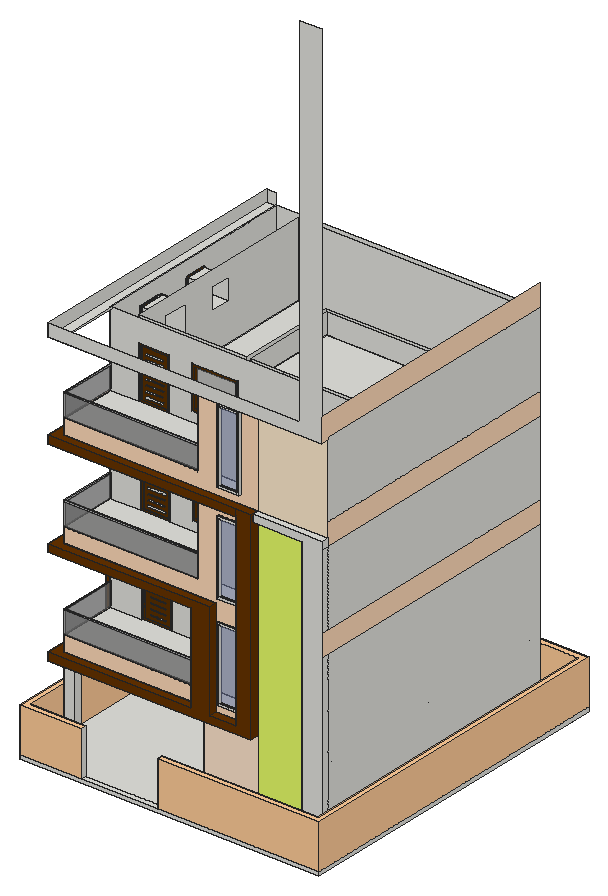
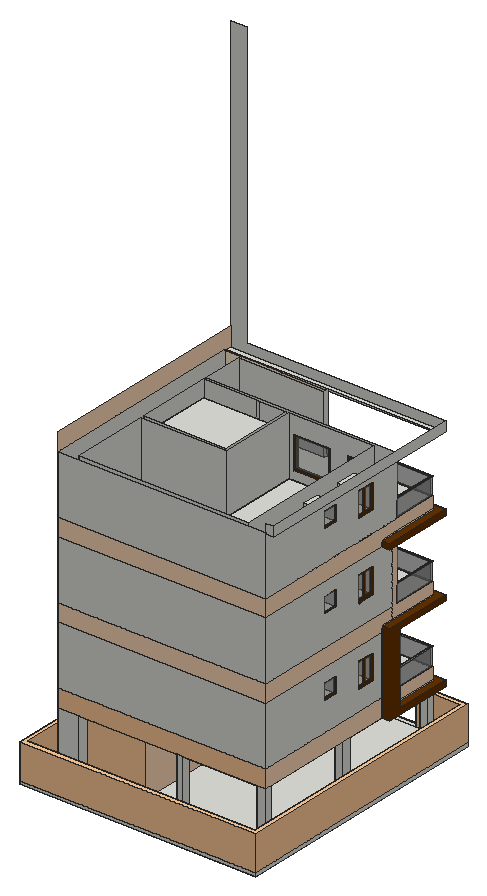
# SketchUp Ruby script. Lengths in inches.
U = 1.inch
M = Sketchup.active_model
def pt(a) = Geom::Point3d.new(a.map { |v| v * U })
def face(e, loops, mat)
  f = e.add_face(loops[0].map { |a| pt(a) })
  loops[1..].each { |l| e.add_face(l.map { |a| pt(a) }).erase! }
  f.material = f.back_material = mat if mat
  f
end
# faces: each face lists its corners as indices into pts; further lists are holes
def faces(e, pts, list, mat = nil) = list.each { |f| face(e, (f[0].is_a?(Array) ? f : [f]).map { |l| l.map { |i| pts[i] } }, mat) }
# xy, xz, yz: faces in a plane at the given z, y or x. An outline is a flat list of corners, or four numbers for a rectangle; further outlines are holes
def ring(l) = l.size == 4 ? [[l[0], l[1]], [l[2], l[1]], [l[2], l[3]], [l[0], l[3]]] : l.each_slice(2).to_a
def flat(e, list, mat, &to3) = list.each { |f| face(e, (f[0].is_a?(Array) ? f : [f]).map { |l| ring(l).map { |u, v| to3.(u, v) } }, mat) }
def xy(e, z, list, mat = nil) = flat(e, list, mat) { |x, y| [x, y, z] }
def xz(e, y, list, mat = nil) = flat(e, list, mat) { |x, z| [x, y, z] }
def yz(e, x, list, mat = nil) = flat(e, list, mat) { |y, z| [x, y, z] }
def lines(e, pts, list) = list.each { |a, b| e.add_line(pt(pts[a]), pt(pts[b])) }
# prism: a flat outline (further loops are holes) pulled along v
def prism(e, loops, v, mat = nil)
  f = face(e, loops, mat); d = Geom::Vector3d.new(v.map { |x| x * U })
  f.pushpull(f.normal.samedirection?(d) ? d.length : -d.length)
end
def box(e, o, s, mat = nil) = prism(e, [[o, [o[0] + s[0], o[1], o[2]], [o[0] + s[0], o[1] + s[1], o[2]], [o[0], o[1] + s[1], o[2]]]], [0, 0, s[2]], mat)
def at(x, y, z, deg = 0) = Geom::Transformation.translation(pt([x, y, z])) * Geom::Transformation.rotation(ORIGIN, Z_AXIS, deg.degrees)
def axes(o, x, y, z) = Geom::Transformation.new([*x, 0, *y, 0, *z, 0, *pt(o).to_a, 1])
def part(name) = M.definitions.add(name)
# library, detail: a bought-in or finely detailed component or shape, given as its bounding box
def library(name, o, s) = part(name).tap { |d| box(d.entities, o, s) }
def detail(e, o, s) = box(e.add_group.entities, o, s)
def put(e, d, t, mat = nil) = e.add_instance(d, t).tap { |i| i.material = mat if mat }
def group(e, t, mat = nil) = e.add_group.tap { |g| g.transformation = t; g.material = mat if mat }.entities
root = M.entities
M.materials.add("[0027_PeachPuff]").color = [255, 218, 185]
M.materials.add("[0029_BlanchedAlmond]").color = [255, 235, 205]
M.materials.add("[Aluminum]").color = [179, 179, 179]
M.materials.add("[Color A08]").color = [89, 48, 0]
M.materials.add("[Color C01]").color = [255, 229, 204]
M.materials.add("[Color C02]").color = [255, 204, 153]
M.materials.add("[Color C08]").color = [102, 51, 0]
M.materials.add("[Color M00]").color = [255, 255, 255]
M.materials.add("[Rectangles Running 4x1]").color = [231, 255, 106]
M.materials.add("[Translucent Glass Gray]").color = [128, 128, 128]
M.materials["[Translucent Glass Gray]"].alpha = 0.5
M.materials.add("[Translucent Glass Sky Reflection]").color = [126, 138, 183]
M.materials["[Translucent Glass Sky Reflection]"].alpha = 0.52
c1 = part("Group\#2")
xy(c1.entities,0,[[0,0,48,6.0625]],"[Color A08]")
xy(c1.entities,2.37,[[2.37,2.1875,45.63,6.0625]])
xy(c1.entities,2.37,[[2.37,0,45.63,2.1875]],"[Color A08]")
xy(c1.entities,81.63,[[2.37,2.1875,45.63,6.0625]])
xy(c1.entities,81.63,[[2.37,0,45.63,2.1875]],"[Color A08]")
xy(c1.entities,84,[[0,0,48,6.0625]],"[Color A08]")
xz(c1.entities,0,[[[0,0,48,84],[2.37,2.37,45.63,81.63]]],"[Color A08]")
xz(c1.entities,2.1875,[[9.64,6.54,37.83,9.91],[9.64,15.35,37.83,18.72],[9.64,24.16,37.83,27.54],[9.64,32.97,37.83,36.35],[9.64,41.79,37.83,45.16],
  [9.64,50.6,37.83,53.97],[9.64,59.41,37.83,62.79],[9.64,68.22,37.83,71.6]])
xz(c1.entities,2.1875,[[[2.37,2.37,45.63,81.63],[9.64,68.22,37.83,71.6],[9.64,59.41,37.83,62.79],[9.64,50.6,37.83,53.97],[9.64,41.79,37.83,45.16],[9.64,32.97,37.83,36.35],[9.64,24.16,37.83,27.54],[9.64,15.35,37.83,18.72],[9.64,6.54,37.83,9.91]]],"[Color A08]")
xz(c1.entities,6.0625,[[[0,0,48,84],[2.37,2.37,45.63,81.63]],[2.37,2.37,45.63,81.63]],"[Color A08]")
yz(c1.entities,0,[[0,0,6.0625,84]],"[Color A08]")
yz(c1.entities,2.37,[[2.1875,2.37,6.0625,81.63]])
yz(c1.entities,2.37,[[0,2.37,2.1875,81.63]],"[Color A08]")
yz(c1.entities,45.63,[[2.1875,2.37,6.0625,81.63]])
yz(c1.entities,45.63,[[0,2.37,2.1875,81.63]],"[Color A08]")
yz(c1.entities,48,[[0,0,6.0625,84]],"[Color A08]")
c2 = part("Group\#1")
xy(c2.entities,0,[[0,0,54.25,4.125]],"[Color A08]")
xy(c2.entities,2.45,[[2.45,0,51.8,4.125]],"[Color A08]")
xy(c2.entities,43.87,[[2.45,0,51.8,4.125]],"[Color A08]")
xy(c2.entities,46.3125,[[0,0,54.25,4.125]],"[Color A08]")
xz(c2.entities,0,[[[0,0,54.25,46.3125],[2.45,2.45,51.8,43.87]]],"[Color A08]")
xz(c2.entities,4.125,[[[0,0,54.25,46.3125],[2.45,2.45,51.8,43.87]]],"[Color A08]")
xz(c2.entities,4.125,[[2.45,2.45,51.8,43.87]],"[Translucent Glass Gray]")
yz(c2.entities,0,[[0,0,4.125,46.3125]],"[Color A08]")
yz(c2.entities,2.45,[[0,2.45,4.125,43.87]],"[Color A08]")
yz(c2.entities,51.8,[[0,2.45,4.125,43.87]],"[Color A08]")
yz(c2.entities,54.25,[[0,0,4.125,46.3125]],"[Color A08]")
c3 = part("Group\#3")
xy(c3.entities,0,[[0,0,1.5,39.25],[1.5,0,2.8125,39.25]],"[Color A08]")
xy(c3.entities,3.22,[[0,3.22,1.5,19.0625],[1.5,3.22,2.8125,19.0625],[1.5,19.0625,2.8125,22.29],[0,22.29,1.5,36.03],[1.5,22.29,2.8125,36.03]],"[Color A08]")
xy(c3.entities,36.03,[[0,3.22,1.5,19.0625],[1.5,3.22,2.8125,19.0625],[0,19.0625,1.5,22.29],[1.5,19.0625,2.8125,22.29],[0,22.29,1.5,36.03],
  [1.5,22.29,2.8125,36.03]],"[Color A08]")
xy(c3.entities,39.25,[[0,0,1.5,39.25],[1.5,0,2.8125,39.25]],"[Color A08]")
xz(c3.entities,0,[[0,0,1.5,39.25],[1.5,0,2.8125,39.25]],"[Color A08]")
xz(c3.entities,3.22,[[0,3.22,1.5,36.03],[1.5,3.22,2.8125,36.03]],"[Color A08]")
xz(c3.entities,19.0625,[[0,3.22,1.5,36.03],[1.5,3.22,2.8125,36.03]],"[Color A08]")
xz(c3.entities,22.29,[[0,3.22,1.5,36.03],[1.5,3.22,2.8125,36.03]],"[Color A08]")
xz(c3.entities,36.03,[[0,3.22,1.5,36.03],[1.5,3.22,2.8125,36.03]],"[Color A08]")
xz(c3.entities,39.25,[[0,0,1.5,39.25],[1.5,0,2.8125,39.25]],"[Color A08]")
yz(c3.entities,0,[[[0,0,39.25,39.25],[3.22,3.22,19.0625,36.03],[22.29,3.22,36.03,36.03]]],"[Color A08]")
yz(c3.entities,1.5,[[[0,0,39.25,39.25],[3.22,3.22,36.03,36.03]],[19.0625,3.22,22.29,36.03]],"[Color A08]")
yz(c3.entities,1.5,[[3.22,3.22,19.0625,36.03],[22.29,3.22,36.03,36.03]],"[Translucent Glass Gray]")
yz(c3.entities,2.8125,[[[0,0,39.25,39.25],[3.22,3.22,36.03,36.03]],[19.0625,3.22,22.29,36.03]],"[Color A08]")
c4 = part("Group\#4")
xy(c4.entities,0,[[0,0,1.5,39.25],[1.5,0,2.8125,39.25]],"[Color A08]")
xy(c4.entities,3.22,[[0,3.22,1.5,36.03],[1.5,3.22,2.8125,36.03]],"[Color A08]")
xy(c4.entities,36.03,[[0,3.22,1.5,36.03],[1.5,3.22,2.8125,36.03]],"[Color A08]")
xy(c4.entities,39.25,[[0,0,1.5,39.25],[1.5,0,2.8125,39.25]],"[Color A08]")
xz(c4.entities,0,[[0,0,1.5,39.25],[1.5,0,2.8125,39.25]],"[Color A08]")
xz(c4.entities,3.22,[[0,3.22,1.5,36.03],[1.5,3.22,2.8125,36.03]],"[Color A08]")
xz(c4.entities,36.03,[[0,3.22,1.5,36.03],[1.5,3.22,2.8125,36.03]],"[Color A08]")
xz(c4.entities,39.25,[[0,0,1.5,39.25],[1.5,0,2.8125,39.25]],"[Color A08]")
yz(c4.entities,0,[[[0,0,39.25,39.25],[3.22,3.22,36.03,36.03]]],"[Color A08]")
yz(c4.entities,1.5,[[[0,0,39.25,39.25],[3.22,3.22,36.03,36.03]]],"[Color A08]")
yz(c4.entities,1.5,[[3.22,3.22,36.03,36.03]],"[Translucent Glass Gray]")
yz(c4.entities,2.8125,[[[0,0,39.25,39.25],[3.22,3.22,36.03,36.03]]],"[Color A08]")
xy(root,0,[[0,0,480,540]],"[Color M00]")
xy(root,6,[[0,0,0,540,480,540,480,0,220.15,0,220.15,9,471,9,471,531,9,531,9,9,98.15,9,98.15,0],[98.15,0,220.15,9],[[9,9,471,531],[414.23,46.6875,414.23,57,249.82,57,249.82,63,417,63,417,251.76,287.75,251.76,287.75,461.375,406.24,461.375,406.24,483,448.4375,483,448.4375,46.6875],[24.5,270.1,42.53,286.06],[24.5,57,42.53,69.13],[24.5,471.06,42.53,483],[193.7,468.4375,207.02,483]],[414.23,46.6875,448.4375,57],[24.5,57,42.53,69.13],
  [249.82,57,249.82,63,417,63,417,251.76,448.4375,251.76,448.4375,57],[[287.75,251.76,448.4375,461.375],[293.77,257.79,417,374.99]],[293.77,257.79,417,374.99],[24.5,270.1,42.53,286.06],[406.24,461.375,448.4375,483],
  [193.7,468.4375,207.02,483],[24.5,471.06,42.53,483]])
xy(root,78,[[0,0,98.15,0,98.15,9,9,9,9,531,471,531,471,9,220.15,9,220.15,0,480,0,480,540,0,540]],"[Color C02]")
xy(root,120,[[293.77,257.79,417,374.99]])
xy(root,126,[[24.5,57,42.53,69.13],[42.53,57,42.53,69.13,24.5,69.13,24.5,270.1,42.53,270.1,42.53,286.06,24.5,286.06,24.5,471.06,42.53,471.06,42.53,483,193.7,483,193.7,468.4375,207.02,468.4375,207.02,483,406.24,483,406.24,461.375,287.75,461.375,287.75,251.76,417,251.76,417,63,249.82,63,249.82,57],[287.75,251.76,293.77,461.375],[293.77,251.76,410.98,257.79],[293.77,257.79,417,374.99],
  [24.5,270.1,42.53,286.06],[293.77,374.99,302.09,461.375],[302.09,374.99,410.98,461.375],[410.98,374.99,417,461.375],[406.24,461.375,410.98,483],
  [410.98,461.375,417,483],[193.7,468.4375,207.02,483],[24.5,471.06,42.53,483]])
xy(root,126,[[9.1875,43.625,9.1875,69.13,24.5,69.13,24.5,57,335.42,57,335.42,43.625],[9.1875,69.13,24.5,187.1]],"[Color C08]")
xy(root,138,[[9.1875,43.625,239.3125,43.625,239.3125,57,24.5,57,24.5,160.8,9.1875,160.8],[268.87,43.625,310.94,57]],"[Color C08]")
xy(root,149.86,[[273.13,54,307.66,57]])
xy(root,152.91,[[276.18,54,304.61,57]])
xy(root,162,[[24.5,57,24.5,149.375,26.5,149.375,26.5,59,239.3125,59,239.3125,57],[26.5,59,239.3125,59,239.3125,66,414,66,414,149.375,123.74,149.375,123.74,155.375,75.74,155.375,75.74,149.375,26.5,149.375],[66,155.375,239.3125,155.375,239.3125,314.6875,414,314.6875,414,474,66,474],[245.3125,155.375,414,308.6875]])
xy(root,179.21,[[157.83,149.375,231.58,155.375]])
xy(root,198,[[24.5,57,24.5,149.375,26.5,149.375,26.5,59,239.3125,59,239.3125,57]],"[Aluminum]")
xy(root,200,[[24.5,57,239.3125,57,239.3125,59,26.5,59,26.5,149.375,24.5,149.375]],"[Aluminum]")
xy(root,202.95,[[24.5,208.14,66,249.33]])
xy(root,220.36,[[24.5,301.46,66,335.96]])
xy(root,246,[[75.74,149.375,123.74,155.375]])
xy(root,247.4,[[157.83,149.375,231.58,155.375]])
xy(root,254.86,[[24.5,301.46,66,335.96]])
xy(root,256.82,[[24.5,208.14,66,249.33]])
xy(root,265.97,[[276.18,54,277.97,57],[277.97,54,280.16,57],[280.16,54,304.61,57]])
xy(root,269.02,[[273.13,54,307.66,57]])
xy(root,282,[[24.5,57,24.5,149.375,414,149.375,414,66,239.3125,66,239.3125,57]])
xy(root,282,[[9.1875,43.625,9.1875,160.8,24.5,160.8,24.5,57,239.3125,57,239.3125,43.625]],"[Color C08]")
xy(root,294,[[9.1875,43.625,268.87,43.625,268.87,57,24.5,57,24.5,187.1,9.1875,187.1]],"[Color C08]")
xy(root,303.05,[[273.13,54,307.66,57]])
xy(root,306.1,[[276.18,54,277.97,57],[277.97,54,304.61,57]])
xy(root,312,[[66,155.375,66,474,414,474,414,314.6875,239.3125,314.6875,239.3125,155.375]])
xy(root,318,[[24.5,57,24.5,149.375,26.5,149.375,26.5,59,239.3125,59,239.3125,57],[26.5,59,239.3125,59,239.3125,66,414,66,414,149.375,121.24,149.375,121.24,155.375,73.24,155.375,73.24,149.375,26.5,149.375],[121.24,149.375,414,155.375],[66,155.375,239.3125,155.375,239.3125,314.6875,414,314.6875,414,474,66,474],[245.3125,155.375,414,308.6875]])
xy(root,325.5625,[[245.3125,155.375,414,308.6875]])
xy(root,332.27,[[156.77,149.375,230.52,155.375]])
xy(root,354,[[24.5,57,24.5,149.375,26.5,149.375,26.5,59,239.3125,59,239.3125,57]],"[Aluminum]")
xy(root,356,[[24.5,57,239.3125,57,239.3125,59,26.5,59,26.5,149.375,24.5,149.375]],"[Aluminum]")
xy(root,360.82,[[24.5,208.14,66,249.33]])
xy(root,378.92,[[24.5,301.46,66,335.96]])
xy(root,400.46,[[156.77,149.375,230.52,155.375]])
xy(root,402,[[73.24,149.375,121.24,155.375]])
xy(root,413.42,[[24.5,301.46,66,335.96]])
xy(root,414.7,[[24.5,208.14,66,249.33]])
xy(root,419.16,[[276.18,54,277.97,57],[277.97,54,280.16,57],[280.16,54,304.61,57]])
xy(root,422.21,[[273.13,54,307.66,57]],"[0027_PeachPuff]")
xy(root,438,[[335.42,46.6875,414.23,57],[24.5,57,24.5,149.375,414,149.375,414,66,239.3125,66,239.3125,57]])
xy(root,438,[[9.1875,43.625,9.1875,187.1,24.5,187.1,24.5,57,239.3125,57,239.3125,43.625],[239.3125,43.625,310.94,57]],"[Color C08]")
xy(root,450,[[335.42,46.6875,448.4375,57]])
xy(root,450,[[9.1875,43.625,335.42,43.625,335.42,57,24.5,57,24.5,187.1,9.1875,187.1]],"[Color C08]")
xy(root,463.11,[[273.13,54,307.66,57]])
xy(root,466.16,[[276.18,54,304.61,57]])
xy(root,468,[[66,155.375,66,474,414,474,414,314.6875,239.3125,314.6875,239.3125,155.375]])
xy(root,474,[[24.5,57,24.5,149.375,26.5,149.375,26.5,59,239.3125,59,239.3125,57],[26.5,59,239.3125,59,239.3125,66,414,66,414,149.375,119.3,149.375,119.3,155.375,71.3,155.375,71.3,149.375,26.5,149.375],[66,155.375,239.3125,155.375,239.3125,314.6875,414,314.6875,414,474,66,474],[245.3125,155.375,414,308.6875]])
xy(root,480,[[245.3125,155.375,414,308.6875]])
xy(root,490.83,[[156.58,149.375,230.33,155.375]])
xy(root,510,[[24.5,57,24.5,149.375,26.5,149.375,26.5,59,239.3125,59,239.3125,57]],"[Aluminum]")
xy(root,512,[[24.5,57,239.3125,57,239.3125,59,26.5,59,26.5,149.375,24.5,149.375]],"[Aluminum]")
xy(root,515.2,[[24.5,208.14,66,249.33]])
xy(root,535.23,[[24.5,301.46,66,335.96]])
xy(root,558,[[71.3,149.375,119.3,155.375]])
xy(root,559.02,[[156.58,149.375,230.33,155.375]])
xy(root,560.8125,[[245.3125,155.375,414,308.6875]])
xy(root,569.07,[[24.5,208.14,66,249.33]])
xy(root,569.73,[[24.5,301.46,66,335.96]])
xy(root,579.22,[[276.18,54,277.97,57],[277.97,54,280.16,57],[280.16,54,283.28,57],[283.28,54,304.61,57]])
xy(root,582.27,[[273.13,54,307.66,57]])
xy(root,591.9375,[[9.1875,43.625,9.1875,483,24.5,483,24.5,149.375,27.5,149.375,27.5,57,448.4375,57,448.4375,43.625]])
xz(root,0,[[0,0,480,6]])
xz(root,0,[[0,6,98.15,78],[220.15,6,480,78]],"[Color C02]")
xz(root,9,[[9,6,98.15,78],[220.15,6,471,78]],"[Color C02]")
xz(root,43.625,[[9.1875,591.9375,448.4375,591.9375,448.4375,1188.8,414.23,1188.8,414.23,611.375,9.1875,611.375]])
xz(root,43.625,[[9.1875,126,335.42,126,335.42,450,310.94,450,310.94,138,268.87,138,268.87,294,9.1875,294,9.1875,282,239.3125,282,239.3125,138,9.1875,138],[9.1875,438,310.94,450]],"[Color C08]")
xz(root,46.6875,[[414.23,6,448.4375,6,448.4375,450,335.42,450,335.42,438,414.23,438]])
xz(root,54,[[[273.13,149.86,307.66,269.02],[276.18,152.91,304.61,265.97]],[[273.13,303.05,307.66,422.21],[276.18,306.1,304.61,419.16]],[[273.13,463.11,307.66,582.27],[276.18,466.16,304.61,579.22]]])
xz(root,57,[[24.5,6,42.53,126],[24.5,126,24.5,138,239.3125,138,239.3125,282,24.5,282,24.5,294,268.87,294,268.87,138,310.94,138,310.94,438,268.87,438,268.87,450,335.42,450,335.42,126],[[273.13,149.86,307.66,269.02],[276.18,152.91,304.61,265.97]],[[273.13,303.05,307.66,422.21],[276.18,306.1,304.61,419.16]],[24.5,438,268.87,450],
  [[273.13,463.11,307.66,582.27],[276.18,466.16,304.61,579.22]],[27.5,591.9375,239.3125,594],[239.3125,591.9375,335.42,594],[335.42,591.9375,414.23,594],[414.23,591.9375,448.4375,594]])
xz(root,57,[[24.5,138,239.3125,162],[[268.87,138,310.94,138,310.94,438,239.3125,438,239.3125,318,24.5,318,24.5,294,268.87,294],[273.13,303.05,307.66,422.21],[273.13,149.86,307.66,269.02]],[[24.5,450,335.42,450,335.42,591.9375,239.3125,591.9375,239.3125,474,24.5,474],[273.13,463.11,307.66,582.27]]],"[0027_PeachPuff]")
xz(root,57,[[335.42,450,448.4375,591.9375]],"[0029_BlanchedAlmond]")
xz(root,57,[[24.5,198,239.3125,200],[24.5,354,239.3125,356],[24.5,510,239.3125,512]],"[Aluminum]")
xz(root,57,[[249.82,6,335.42,126]],"[Color C01]")
xz(root,57,[[335.42,6,414.23,438]],"[Rectangles Running 4x1]")
xz(root,57,[[24.5,162,239.3125,198],[24.5,318,239.3125,354],[24.5,474,239.3125,510]],"[Translucent Glass Gray]")
xz(root,57,[[276.18,152.91,304.61,265.97],[276.18,306.1,304.61,419.16],[276.18,466.16,304.61,579.22]],"[Translucent Glass Sky Reflection]")
xz(root,59,[[26.5,198,239.3125,200],[26.5,354,239.3125,356],[26.5,510,239.3125,512]],"[Aluminum]")
xz(root,59,[[26.5,162,239.3125,198],[26.5,318,239.3125,354],[26.5,474,239.3125,510]],"[Translucent Glass Gray]")
xz(root,63,[[249.82,6,417,126]])
xz(root,66,[[239.3125,162,414,282],[239.3125,318,414,438],[239.3125,474,414,594]])
xz(root,69.13,[[24.5,6,42.53,126]])
xz(root,149.375,[[24.5,162,26.5,198],[[26.5,162,75.74,162,75.74,246,123.74,246,123.74,162,414,162,414,282,24.5,282,24.5,200,26.5,200],[157.83,179.21,231.58,247.4]],[239.3125,282,414,318],[24.5,318,26.5,354],[[26.5,318,73.24,318,73.24,402,121.24,402,121.24,318,414,318,414,438,24.5,438,24.5,356,26.5,356],[156.77,332.27,230.52,400.46]],
  [239.3125,438,414,474],[24.5,474,26.5,510],[[26.5,474,71.3,474,71.3,558,119.3,558,119.3,474,414,474,414,594,27.5,594,27.5,591.9375,24.5,591.9375,24.5,512,26.5,512],[156.58,490.83,230.33,559.02]],[24.5,591.9375,27.5,594]])
xz(root,149.375,[[24.5,198,26.5,200],[24.5,354,26.5,356],[24.5,510,26.5,512]],"[Aluminum]")
xz(root,155.375,[[[66,162,66,282,239.3125,282,239.3125,162,123.74,162,123.74,246,75.74,246,75.74,162],[157.83,179.21,231.58,247.4]],[245.3125,162,414,282],[66,282,239.3125,312],[245.3125,282,414,318],[66,312,73.24,318],
  [73.24,312,121.24,318],[121.24,312,227.8125,318],[227.8125,312,239.3125,318],[[66,318,66,438,239.3125,438,239.3125,318,121.24,318,121.24,402,73.24,402,73.24,318],[156.77,332.27,230.52,400.46]],[245.3125,318,389.91,325.5625],
  [389.91,318,401.23,325.5625],[401.23,318,414,325.5625],[245.3125,325.5625,414,438],[66,438,239.3125,468],[245.3125,438,414,474],
  [66,468,71.3,474],[71.3,468,119.3,474],[119.3,468,230.75,474],[230.75,468,239.3125,474],[[66,474,66,594,239.3125,594,239.3125,474,119.3,474,119.3,558,71.3,558,71.3,474],[156.58,490.83,230.33,559.02]],
  [245.3125,474,362.52,480],[362.52,474,370.65,480],[370.65,474,414,480],[245.3125,480,414,560.8125],[245.3125,560.8125,298.66,594],
  [298.66,560.8125,307.22,594],[298.66,560.8125,307.22,594],[307.22,560.8125,414,594]])
xz(root,160.8,[[9.1875,138,24.5,282]],"[Color C08]")
xz(root,187.1,[[9.1875,126,24.5,294],[9.1875,438,24.5,450]],"[Color C08]")
xz(root,208.14,[[24.5,202.95,66,256.82],[24.5,360.82,66,414.7],[24.5,515.2,66,569.07]])
xz(root,249.33,[[24.5,202.95,66,256.82],[24.5,360.82,66,414.7],[24.5,515.2,66,569.07]])
xz(root,251.76,[[287.75,6,417,126]],"[0027_PeachPuff]")
xz(root,257.79,[[293.77,6,410.98,120],[410.98,6,417,120],[293.77,120,410.98,126],[410.98,120,417,126]])
xz(root,270.1,[[24.5,6,42.53,126]])
xz(root,286.06,[[24.5,6,42.53,126]])
xz(root,301.46,[[24.5,220.36,66,254.86],[24.5,378.92,66,413.42],[24.5,535.23,66,569.73]])
xz(root,308.6875,[[245.3125,162,414,282],[245.3125,282,414,318],[245.3125,318,414,325.5625],[245.3125,325.5625,414,438],[245.3125,438,414,474],
  [245.3125,474,414,480],[245.3125,480,414,560.8125],[245.3125,560.8125,414,594]])
xz(root,314.6875,[[239.3125,162,414,282],[239.3125,282,414,312],[239.3125,312,414,318],[239.3125,318,414,438],[239.3125,438,414,468],
  [239.3125,468,414,474],[239.3125,474,414,594]])
xz(root,335.96,[[24.5,220.36,66,254.86],[24.5,378.92,66,413.42],[24.5,535.23,66,569.73]])
xz(root,374.99,[[293.77,6,410.98,120],[410.98,6,417,120],[293.77,120,302.09,126],[302.09,120,410.98,126],[410.98,120,417,126]])
xz(root,461.375,[[287.75,6,406.24,126]],"[Color C02]")
xz(root,468.4375,[[193.7,6,207.02,126]])
xz(root,471.06,[[24.5,6,42.53,126]])
xz(root,474,[[66,162,414,282],[66,282,414,312],[66,312,414,318],[66,318,414,438],[66,438,414,468],
  [66,468,414,474],[66,474,414,594]])
xz(root,483,[[24.5,6,42.53,126],[193.7,6,207.02,126],[406.24,6,448.4375,126],[24.5,162,448.4375,282],[24.5,318,448.4375,438],
  [24.5,474,448.4375,594],[9.1875,591.9375,24.5,611.375]])
xz(root,483,[[24.5,282,448.4375,318],[24.5,438,448.4375,474]],"[0027_PeachPuff]")
xz(root,483,[[24.5,126,448.4375,162]],"[Color C02]")
xz(root,531,[[9,6,471,78]],"[Color C02]")
xz(root,540,[[0,0,480,6]])
xz(root,540,[[0,6,480,78]],"[Color C02]")
yz(root,0,[[0,0,540,6]])
yz(root,0,[[0,6,540,78]],"[Color C02]")
yz(root,9,[[9,6,531,78]],"[Color C02]")
yz(root,9.1875,[[43.625,591.9375,483,611.375]])
yz(root,9.1875,[[43.625,126,43.625,138,160.8,138,160.8,282,43.625,282,43.625,294,187.1,294,187.1,126],[43.625,438,187.1,450]],"[Color C08]")
yz(root,24.5,[[57,6,69.13,126],[270.1,6,286.06,126],[471.06,6,483,126],[57,126,187.1,126,187.1,294,57,294,57,282,160.8,282,160.8,138,57,138],[[187.1,162,483,282],[208.14,202.95,249.33,256.82],[301.46,220.36,335.96,254.86]],
  [[160.8,318,483,438],[208.14,360.82,249.33,414.7],[301.46,378.92,335.96,413.42]],[57,438,160.8,450],[160.8,438,187.1,450],[[149.375,474,483,591.9375],[208.14,515.2,249.33,569.07],[301.46,535.23,335.96,569.73]],[149.375,591.9375,187.1,594],
  [187.1,591.9375,483,594]])
yz(root,24.5,[[187.1,126,483,162],[57,138,57,162,149.375,162,149.375,282,160.8,282,160.8,138],[187.1,282,187.1,294,160.8,294,160.8,318,483,318,483,282],[57,294,57,318,149.375,318,149.375,438,160.8,438,160.8,294],[187.1,438,187.1,450,57,450,57,474,483,474,483,438]],"[0027_PeachPuff]")
yz(root,24.5,[[57,198,149.375,200],[57,354,149.375,356],[57,510,149.375,512]],"[Aluminum]")
yz(root,24.5,[[57,162,149.375,198],[57,318,149.375,354],[57,474,149.375,510]],"[Translucent Glass Gray]")
yz(root,26.5,[[59,198,149.375,200],[59,354,149.375,356],[59,510,149.375,512]],"[Aluminum]")
yz(root,26.5,[[59,162,149.375,198],[59,318,149.375,354],[59,474,149.375,510]],"[Translucent Glass Gray]")
yz(root,27.5,[[57,591.9375,149.375,594]])
yz(root,42.53,[[57,6,69.13,126],[270.1,6,286.06,126],[471.06,6,483,126]])
yz(root,66,[[[155.375,162,474,282],[208.14,202.95,249.33,256.82],[301.46,220.36,335.96,254.86]],[155.375,282,474,312],[155.375,312,474,318],[[155.375,318,474,438],[208.14,360.82,249.33,414.7],[301.46,378.92,335.96,413.42]],[155.375,438,474,468],
  [155.375,468,474,474],[[155.375,474,474,594],[208.14,515.2,249.33,569.07],[301.46,535.23,335.96,569.73]]])
yz(root,71.3,[[149.375,474,155.375,558]])
yz(root,73.24,[[149.375,318,155.375,402]])
yz(root,75.74,[[149.375,162,155.375,246]])
yz(root,98.15,[[0,6,9,78]])
yz(root,119.3,[[149.375,474,155.375,558]])
yz(root,121.24,[[149.375,318,155.375,402]])
yz(root,123.74,[[149.375,162,155.375,246]])
yz(root,156.58,[[149.375,490.83,155.375,559.02]])
yz(root,156.77,[[149.375,332.27,155.375,400.46]])
yz(root,157.83,[[149.375,179.21,155.375,247.4]])
yz(root,193.7,[[468.4375,6,483,126]])
yz(root,207.02,[[468.4375,6,483,126]])
yz(root,220.15,[[0,6,9,78]],"[Color C02]")
yz(root,230.33,[[149.375,490.83,155.375,559.02]])
yz(root,230.52,[[149.375,332.27,155.375,400.46]])
yz(root,231.58,[[149.375,179.21,155.375,247.4]])
yz(root,239.3125,[[57,162,59,198],[155.375,162,314.6875,282],[155.375,282,314.6875,312],[155.375,312,314.6875,318],[57,318,59,354],
  [59,318,59,356,57,356,57,438,66,438,66,318],[155.375,318,314.6875,438],[155.375,438,314.6875,468],[155.375,468,314.6875,474],[57,474,59,510],
  [59,474,59,512,57,512,57,594,66,594,66,474],[155.375,474,314.6875,594]])
yz(root,239.3125,[[57,198,59,200],[57,354,59,356],[57,510,59,512]],"[Aluminum]")
yz(root,239.3125,[[59,162,59,200,57,200,57,282,66,282,66,162]],"[Color C01]")
yz(root,239.3125,[[43.625,138,57,282]],"[Color C08]")
yz(root,245.3125,[[155.375,162,308.6875,282],[155.375,282,308.6875,318],[155.375,318,308.6875,325.5625],[155.375,325.5625,308.6875,438],[155.375,438,308.6875,474],
  [155.375,474,308.6875,480],[155.375,480,308.6875,560.8125],[155.375,560.8125,308.6875,594]])
yz(root,249.82,[[57,6,63,126]],"[Color C01]")
yz(root,268.87,[[43.625,138,57,294]],"[Color C08]")
yz(root,273.13,[[54,149.86,57,269.02],[54,303.05,57,422.21],[54,463.11,57,582.27]])
yz(root,276.18,[[54,152.91,57,265.97],[54,306.1,57,419.16],[54,466.16,57,579.22]])
yz(root,287.75,[[251.76,6,461.375,126]],"[0027_PeachPuff]")
yz(root,293.77,[[257.79,6,374.99,120],[257.79,120,374.99,126]])
yz(root,304.61,[[54,152.91,57,265.97],[54,306.1,57,419.16],[54,466.16,57,579.22]])
yz(root,307.66,[[54,149.86,57,269.02],[54,303.05,57,422.21],[54,463.11,57,582.27]])
yz(root,310.94,[[43.625,138,57,438]],"[Color C08]")
yz(root,335.42,[[46.6875,438,57,450]])
yz(root,335.42,[[43.625,126,57,126,57,438,46.6875,438,46.6875,450,43.625,450]],"[Color C08]")
yz(root,406.24,[[461.375,6,483,126]])
yz(root,414,[[66,162,149.375,282],[155.375,162,308.6875,282],[314.6875,162,474,282],[66,282,149.375,318],[149.375,282,155.375,318],
  [155.375,282,308.6875,318],[314.6875,282,474,312],[314.6875,312,474,318],[66,318,149.375,438],[155.375,318,308.6875,325.5625],
  [314.6875,318,474,438],[155.375,325.5625,308.6875,438],[66,438,149.375,474],[155.375,438,308.6875,474],[314.6875,438,474,468],
  [314.6875,468,474,474],[66,474,149.375,594],[155.375,474,308.6875,480],[314.6875,474,474,594],[155.375,480,308.6875,560.8125],
  [155.375,560.8125,308.6875,594]])
yz(root,414.23,[[46.6875,6,57,438]])
yz(root,417,[[63,6,251.76,126],[257.79,6,374.99,120],[257.79,120,374.99,126]])
yz(root,448.4375,[[46.6875,6,57,282],[57,6,483,282],[46.6875,318,57,438],[57,318,483,438],[46.6875,438,57,450],
  [57,474,483,594]])
yz(root,448.4375,[[46.6875,282,483,318],[57,438,483,474],[43.625,591.9375,57,591.9375,57,594,483,594,483,630,43.625,630]],"[0027_PeachPuff]")
yz(root,471,[[9,6,531,78]],"[Color C02]")
yz(root,480,[[0,0,540,6]])
yz(root,480,[[0,6,540,78]],"[Color C02]")
p = [[410.98,63,126],[410.98,57,126],[417,257.79,126],[448.4375,257.79,126],[417,63,126],[448.4375,63,126],
  [448.4375,461.375,126],[417,461.375,126],[239.3125,155.375,282],[245.3125,155.375,282],[239.3125,66,318],[239.3125,66,282],
  [239.3125,66,438],[239.3125,66,474],[239.3125,57,474],[239.3125,57,471.72]]
lines(root,p,[[0,1],[2,3],[4,5],[6,7],[8,9],[10,11],[12,13],[14,15]])
put(root,c1,at(75.74,150.25,162))
put(root,c2,axes([157.83,149.375,179.21],[1.35945,0,0],[0,1,0],[0,0,1.47233]))
put(root,c3,axes([26.1875,208.14,202.95],[1,0,0],[0,1.04,0],[0,0,1.3635]))
put(root,c4,axes([26.7,301.46,220.36],[0.78,0,0],[0,0.897,0],[0,0,0.88312]))
put(root,c1,at(73.24,150.25,318))
put(root,c2,axes([156.77,149.375,332.27],[1.35945,0,0],[0,1,0],[0,0,1.47233]))
put(root,c3,axes([26.1875,208.14,360.82],[1,0,0],[0,1.04,0],[0,0,1.3635]))
put(root,c4,axes([25.12,301.46,378.92],[0.78,0,0],[0,0.897,0],[0,0,0.88312]))
put(root,c1,at(71.3,149.375,474))
put(root,c2,axes([156.58,149.375,490.83],[1.35945,0,0],[0,1,0],[0,0,1.47233]))
put(root,c3,axes([26.1875,208.14,515.2],[1,0,0],[0,1.04,0],[0,0,1.3635]))
put(root,c4,axes([25.12,301.46,535.23],[0.78,0,0],[0,0.897,0],[0,0,0.88312]))
